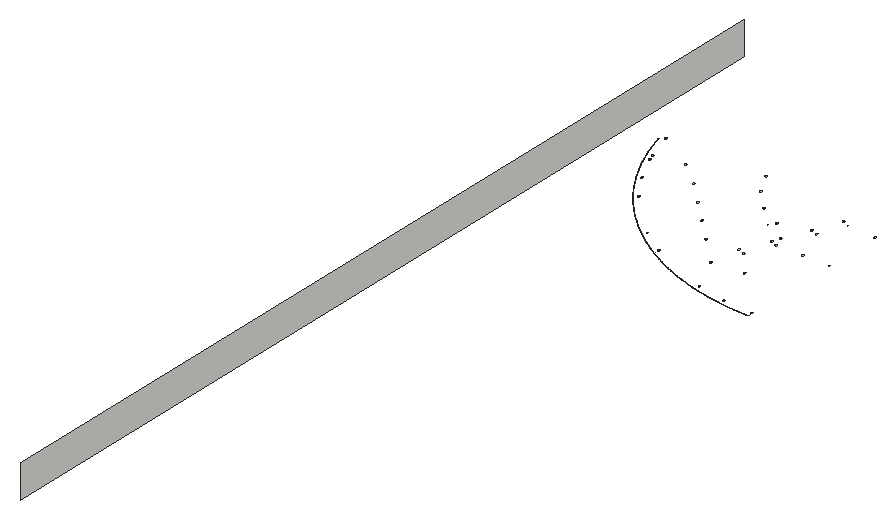
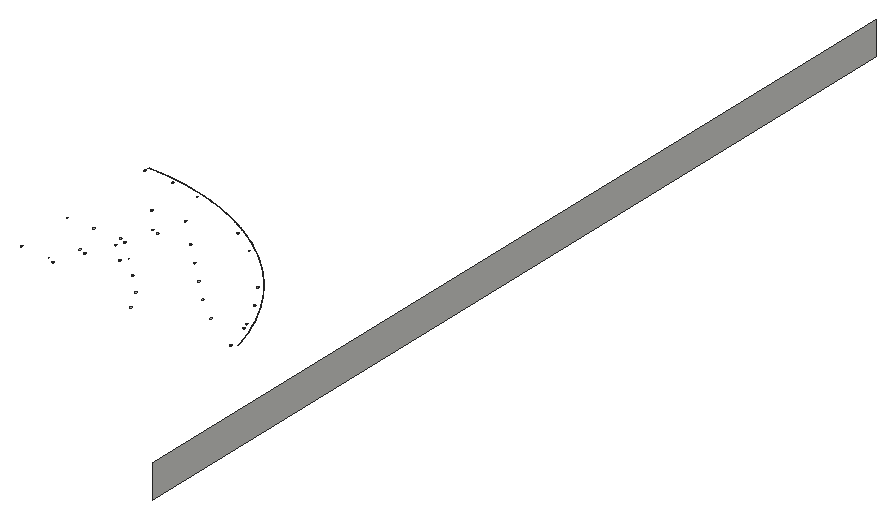
# SketchUp Ruby script. Lengths in inches.
U = 1.inch
M = Sketchup.active_model
def pt(a) = Geom::Point3d.new(a.map { |v| v * U })
def face(e, loops, mat)
  f = e.add_face(loops[0].map { |a| pt(a) })
  loops[1..].each { |l| e.add_face(l.map { |a| pt(a) }).erase! }
  f.material = f.back_material = mat if mat
  f
end
# faces: each face lists its corners as indices into pts; further lists are holes
def faces(e, pts, list, mat = nil) = list.each { |f| face(e, (f[0].is_a?(Array) ? f : [f]).map { |l| l.map { |i| pts[i] } }, mat) }
# xy, xz, yz: faces in a plane at the given z, y or x. An outline is a flat list of corners, or four numbers for a rectangle; further outlines are holes
def ring(l) = l.size == 4 ? [[l[0], l[1]], [l[2], l[1]], [l[2], l[3]], [l[0], l[3]]] : l.each_slice(2).to_a
def flat(e, list, mat, &to3) = list.each { |f| face(e, (f[0].is_a?(Array) ? f : [f]).map { |l| ring(l).map { |u, v| to3.(u, v) } }, mat) }
def xy(e, z, list, mat = nil) = flat(e, list, mat) { |x, y| [x, y, z] }
def xz(e, y, list, mat = nil) = flat(e, list, mat) { |x, z| [x, y, z] }
def yz(e, x, list, mat = nil) = flat(e, list, mat) { |y, z| [x, y, z] }
def lines(e, pts, list) = list.each { |a, b| e.add_line(pt(pts[a]), pt(pts[b])) }
# prism: a flat outline (further loops are holes) pulled along v
def prism(e, loops, v, mat = nil)
  f = face(e, loops, mat); d = Geom::Vector3d.new(v.map { |x| x * U })
  f.pushpull(f.normal.samedirection?(d) ? d.length : -d.length)
end
def box(e, o, s, mat = nil) = prism(e, [[o, [o[0] + s[0], o[1], o[2]], [o[0] + s[0], o[1] + s[1], o[2]], [o[0], o[1] + s[1], o[2]]]], [0, 0, s[2]], mat)
def at(x, y, z, deg = 0) = Geom::Transformation.translation(pt([x, y, z])) * Geom::Transformation.rotation(ORIGIN, Z_AXIS, deg.degrees)
def axes(o, x, y, z) = Geom::Transformation.new([*x, 0, *y, 0, *z, 0, *pt(o).to_a, 1])
def part(name) = M.definitions.add(name)
# library, detail: a bought-in or finely detailed component or shape, given as its bounding box
def library(name, o, s) = part(name).tap { |d| box(d.entities, o, s) }
def detail(e, o, s) = box(e.add_group.entities, o, s)
def put(e, d, t, mat = nil) = e.add_instance(d, t).tap { |i| i.material = mat if mat }
def group(e, t, mat = nil) = e.add_group.tap { |g| g.transformation = t; g.material = mat if mat }.entities
root = M.entities
M.materials.add("[Asphalt_Stamped_Brick]").color = [149, 133, 134]
M.materials.add("[Metal_Steel_Textured_White]").color = [191, 191, 191]
xy(root,3.625,[[146.528,137.349,146.523,137.35,146.518,137.352,146.514,137.355,146.511,137.359,146.509,137.364,146.508,137.369,146.509,137.374,146.511,137.379,146.514,137.383,146.518,137.387,146.523,137.389,146.533,137.389,146.538,137.387,146.542,137.383,146.545,137.379,146.547,137.374,146.548,137.369,146.547,137.364,146.545,137.359,146.542,137.355,146.538,137.352,146.533,137.35],[143.285,137.968,143.28,137.97,143.276,137.974,143.273,137.978,143.271,137.983,143.27,137.988,143.271,137.993,143.273,137.998,143.276,138.002,143.28,138.005,143.285,138.007,143.29,138.008,143.295,138.007,143.3,138.005,143.304,138.002,143.308,137.998,143.31,137.993,143.31,137.983,143.308,137.978,143.3,137.97,143.295,137.968],[136.475,140.789,136.47,140.791,136.466,140.794,136.463,140.799,136.461,140.803,136.46,140.809,136.461,140.814,136.463,140.819,136.466,140.823,136.47,140.826,136.475,140.828,136.486,140.828,136.49,140.826,136.495,140.823,136.498,140.819,136.5,140.814,136.5,140.803,136.498,140.799,136.495,140.794,136.49,140.791,136.486,140.789],[141.393,141.988,141.388,141.99,141.384,141.993,141.381,141.998,141.379,142.002,141.378,142.008,141.379,142.013,141.381,142.018,141.384,142.022,141.388,142.025,141.393,142.027,141.398,142.028,141.404,142.027,141.408,142.025,141.412,142.022,141.416,142.018,141.418,142.013,141.418,142.002,141.416,141.998,141.412,141.993,141.408,141.99,141.404,141.988],[144.852,142.332,144.847,142.333,144.842,142.335,144.838,142.338,144.834,142.342,144.832,142.347,144.832,142.357,144.834,142.362,144.838,142.366,144.842,142.369,144.847,142.371,144.852,142.372,144.857,142.371,144.862,142.369,144.866,142.366,144.869,142.362,144.871,142.357,144.872,142.352,144.871,142.347,144.869,142.342,144.866,142.338,144.862,142.335,144.857,142.333],
  [133.748,142.641,133.744,142.643,133.736,142.651,133.734,142.656,133.734,142.666,133.736,142.671,133.74,142.675,133.744,142.678,133.748,142.68,133.754,142.681,133.759,142.68,133.764,142.678,133.768,142.675,133.771,142.671,133.773,142.666,133.774,142.661,133.773,142.656,133.771,142.651,133.768,142.647,133.764,142.643,133.759,142.641],[129.101,147.293,129.096,147.294,129.091,147.296,129.087,147.299,129.084,147.303,129.082,147.308,129.081,147.313,129.082,147.318,129.084,147.323,129.087,147.327,129.091,147.33,129.096,147.332,129.101,147.333,129.106,147.332,129.111,147.33,129.115,147.327,129.118,147.323,129.12,147.318,129.121,147.313,129.12,147.308,129.118,147.303,129.115,147.299,129.111,147.296,129.106,147.294],[136.116,147.32,136.111,147.322,136.107,147.326,136.104,147.33,136.102,147.334,136.101,147.34,136.102,147.345,136.104,147.35,136.107,147.354,136.111,147.357,136.116,147.359,136.121,147.36,136.126,147.359,136.131,147.357,136.135,147.354,136.138,147.35,136.14,147.345,136.141,147.34,136.14,147.334,136.138,147.33,136.135,147.326,136.131,147.322,136.126,147.32],[143.146,148.293,143.141,148.294,143.136,148.296,143.132,148.299,143.129,148.303,143.127,148.308,143.126,148.313,143.127,148.318,143.129,148.323,143.132,148.327,143.136,148.33,143.141,148.332,143.146,148.333,143.151,148.332,143.156,148.33,143.16,148.327,143.163,148.323,143.165,148.318,143.166,148.313,143.165,148.308,143.163,148.303,143.16,148.299,143.156,148.296,143.151,148.294],[141.49,151.073,141.485,151.075,141.481,151.079,141.478,151.083,141.476,151.088,141.476,151.098,141.478,151.103,141.481,151.107,141.485,151.11,141.49,151.112,141.495,151.113,141.501,151.112,141.505,151.11,141.51,151.107,141.513,151.103,141.515,151.098,141.515,151.088,141.513,151.083,141.51,151.079,141.505,151.075,141.501,151.073],
  [144.679,151.995,144.674,151.996,144.669,151.998,144.665,152.001,144.662,152.005,144.66,152.01,144.659,152.015,144.66,152.02,144.662,152.025,144.665,152.029,144.669,152.033,144.674,152.035,144.685,152.035,144.689,152.033,144.694,152.029,144.697,152.025,144.699,152.02,144.699,152.01,144.697,152.005,144.694,152.001,144.689,151.998,144.685,151.996],[138.95,152.489,138.945,152.49,138.94,152.492,138.936,152.495,138.932,152.499,138.93,152.504,138.93,152.514,138.932,152.519,138.94,152.527,138.945,152.529,138.955,152.529,138.96,152.527,138.964,152.523,138.967,152.519,138.969,152.514,138.97,152.509,138.969,152.504,138.967,152.499,138.964,152.495,138.96,152.492,138.955,152.49],[125.749,152.958,125.744,152.96,125.74,152.963,125.736,152.968,125.734,152.972,125.734,152.983,125.736,152.988,125.74,152.992,125.744,152.995,125.749,152.997,125.754,152.998,125.759,152.997,125.764,152.995,125.768,152.992,125.771,152.988,125.773,152.983,125.774,152.978,125.773,152.972,125.771,152.968,125.768,152.963,125.764,152.96,125.759,152.958],[125.448,153.695,125.443,153.696,125.438,153.698,125.434,153.701,125.431,153.705,125.429,153.71,125.428,153.715,125.429,153.72,125.431,153.725,125.434,153.729,125.438,153.733,125.443,153.735,125.453,153.735,125.458,153.733,125.462,153.729,125.465,153.725,125.467,153.72,125.468,153.715,125.467,153.71,125.465,153.705,125.462,153.701,125.458,153.698,125.453,153.696],[145.882,154.899,145.877,154.9,145.872,154.902,145.868,154.905,145.865,154.909,145.863,154.914,145.862,154.919,145.863,154.924,145.865,154.929,145.868,154.933,145.872,154.936,145.877,154.938,145.882,154.939,145.887,154.938,145.892,154.936,145.896,154.933,145.9,154.929,145.902,154.924,145.902,154.914,145.9,154.909,145.896,154.905,145.892,154.902,145.887,154.9],
  [124.428,156.83,124.423,156.831,124.418,156.833,124.414,156.836,124.411,156.84,124.409,156.845,124.408,156.85,124.409,156.855,124.411,156.86,124.414,156.864,124.418,156.867,124.423,156.869,124.428,156.87,124.433,156.869,124.438,156.867,124.442,156.864,124.446,156.86,124.448,156.855,124.448,156.845,124.446,156.84,124.442,156.836,124.438,156.833,124.433,156.831]],"[Asphalt_Stamped_Brick]")
xy(root,3.625,[[149.818,137.073,149.795,137.076,149.773,137.085,149.755,137.099,149.741,137.118,149.732,137.139,149.729,137.162,149.732,137.185,149.741,137.207,149.755,137.225,149.773,137.239,149.795,137.248,149.818,137.251,149.818,137.25,149.795,137.247,149.774,137.238,149.756,137.224,149.742,137.206,149.733,137.185,149.73,137.162,149.733,137.139,149.742,137.118,149.756,137.1,149.774,137.086,149.795,137.077,149.818,137.074],[149.818,137.074,149.795,137.077,149.774,137.086,149.756,137.1,149.742,137.118,149.733,137.139,149.73,137.162,149.733,137.185,149.742,137.206,149.756,137.224,149.774,137.238,149.795,137.247,149.818,137.25,149.818,137.199,149.808,137.197,149.8,137.194,149.792,137.188,149.786,137.18,149.783,137.172,149.781,137.162,149.783,137.153,149.786,137.144,149.792,137.136,149.8,137.13,149.808,137.127,149.818,137.125],[149.818,137.125,149.808,137.127,149.8,137.13,149.792,137.136,149.786,137.144,149.783,137.153,149.781,137.162,149.783,137.172,149.786,137.18,149.792,137.188,149.8,137.194,149.808,137.197,149.818,137.199,149.818,137.182,149.813,137.181,149.808,137.179,149.804,137.176,149.801,137.172,149.799,137.167,149.798,137.162,149.799,137.157,149.801,137.152,149.804,137.148,149.808,137.145,149.813,137.143,149.818,137.142],[149.818,137.142,149.818,137.182,149.823,137.181,149.828,137.179,149.832,137.176,149.835,137.172,149.837,137.167,149.838,137.162,149.837,137.157,149.835,137.152,149.832,137.148,149.828,137.145,149.823,137.143],[[146.528,137.281,146.505,137.284,146.484,137.293,146.466,137.307,146.452,137.325,146.443,137.347,146.44,137.369,146.443,137.392,146.452,137.413,146.466,137.432,146.484,137.445,146.505,137.454,146.528,137.457,146.551,137.454,146.572,137.445,146.59,137.432,146.604,137.413,146.613,137.392,146.616,137.369,146.613,137.347,146.604,137.325,146.59,137.307,146.572,137.293,146.551,137.284],[146.528,137.333,146.538,137.334,146.546,137.338,146.554,137.343,146.56,137.351,146.563,137.36,146.565,137.369,146.563,137.379,146.56,137.388,146.554,137.395,146.546,137.401,146.538,137.405,146.528,137.406,146.519,137.405,146.51,137.401,146.502,137.395,146.496,137.388,146.493,137.379,146.491,137.369,146.493,137.36,146.496,137.351,146.502,137.343,146.51,137.338,146.519,137.334]],
  [[146.528,137.333,146.519,137.334,146.51,137.338,146.502,137.343,146.496,137.351,146.493,137.36,146.491,137.369,146.493,137.379,146.496,137.388,146.502,137.395,146.51,137.401,146.519,137.405,146.528,137.406,146.538,137.405,146.546,137.401,146.554,137.395,146.56,137.388,146.563,137.379,146.565,137.369,146.563,137.36,146.56,137.351,146.554,137.343,146.546,137.338,146.538,137.334],[146.528,137.349,146.533,137.35,146.538,137.352,146.542,137.355,146.545,137.359,146.547,137.364,146.548,137.369,146.547,137.374,146.545,137.379,146.542,137.383,146.538,137.387,146.533,137.389,146.523,137.389,146.518,137.387,146.514,137.383,146.511,137.379,146.509,137.374,146.508,137.369,146.509,137.364,146.511,137.359,146.514,137.355,146.518,137.352,146.523,137.35]],[[143.29,137.9,143.268,137.903,143.246,137.912,143.228,137.926,143.214,137.944,143.205,137.965,143.202,137.988,143.205,138.011,143.214,138.032,143.228,138.05,143.246,138.064,143.268,138.073,143.29,138.076,143.313,138.073,143.334,138.064,143.352,138.05,143.366,138.032,143.375,138.011,143.378,137.988,143.375,137.965,143.366,137.944,143.352,137.926,143.334,137.912,143.313,137.903],[143.29,137.951,143.3,137.952,143.309,137.956,143.316,137.962,143.322,137.969,143.326,137.978,143.327,137.988,143.326,137.997,143.322,138.006,143.316,138.014,143.309,138.019,143.3,138.023,143.29,138.024,143.281,138.023,143.272,138.019,143.264,138.014,143.259,138.006,143.255,137.997,143.254,137.988,143.255,137.978,143.259,137.969,143.264,137.962,143.272,137.956,143.281,137.952]],[[143.29,137.951,143.281,137.952,143.272,137.956,143.264,137.962,143.259,137.969,143.255,137.978,143.254,137.988,143.255,137.997,143.259,138.006,143.264,138.014,143.272,138.019,143.281,138.023,143.29,138.024,143.3,138.023,143.309,138.019,143.316,138.014,143.322,138.006,143.326,137.997,143.327,137.988,143.326,137.978,143.322,137.969,143.316,137.962,143.309,137.956,143.3,137.952],[143.285,137.968,143.295,137.968,143.3,137.97,143.308,137.978,143.31,137.983,143.31,137.993,143.308,137.998,143.304,138.002,143.3,138.005,143.295,138.007,143.29,138.008,143.285,138.007,143.28,138.005,143.276,138.002,143.273,137.998,143.271,137.993,143.27,137.988,143.271,137.983,143.273,137.978,143.276,137.974,143.28,137.97]],[[136.48,140.721,136.458,140.724,136.436,140.732,136.418,140.746,136.404,140.765,136.395,140.786,136.392,140.809,136.395,140.831,136.404,140.852,136.418,140.871,136.436,140.885,136.458,140.893,136.48,140.896,136.503,140.893,136.524,140.885,136.543,140.871,136.557,140.852,136.565,140.831,136.568,140.809,136.565,140.786,136.557,140.765,136.543,140.746,136.524,140.732,136.503,140.724],[136.48,140.772,136.49,140.773,136.499,140.777,136.506,140.783,136.512,140.79,136.516,140.799,136.517,140.809,136.516,140.818,136.512,140.827,136.506,140.834,136.499,140.84,136.49,140.844,136.48,140.845,136.471,140.844,136.462,140.84,136.455,140.834,136.449,140.827,136.445,140.818,136.444,140.809,136.445,140.799,136.449,140.79,136.455,140.783,136.462,140.777,136.471,140.773]],[[136.48,140.772,136.471,140.773,136.462,140.777,136.455,140.783,136.449,140.79,136.445,140.799,136.444,140.809,136.445,140.818,136.449,140.827,136.455,140.834,136.462,140.84,136.471,140.844,136.48,140.845,136.49,140.844,136.499,140.84,136.506,140.834,136.512,140.827,136.516,140.818,136.517,140.809,136.516,140.799,136.512,140.79,136.506,140.783,136.499,140.777,136.49,140.773],[136.475,140.789,136.486,140.789,136.49,140.791,136.495,140.794,136.498,140.799,136.5,140.803,136.5,140.814,136.498,140.819,136.495,140.823,136.49,140.826,136.486,140.828,136.475,140.828,136.47,140.826,136.466,140.823,136.463,140.819,136.461,140.814,136.46,140.809,136.461,140.803,136.463,140.799,136.466,140.794,136.47,140.791]],
  [[141.398,141.92,141.376,141.923,141.354,141.931,141.336,141.945,141.322,141.964,141.313,141.985,141.31,142.008,141.313,142.03,141.322,142.052,141.336,142.07,141.354,142.084,141.376,142.093,141.398,142.096,141.421,142.093,141.442,142.084,141.461,142.07,141.474,142.052,141.483,142.03,141.486,142.008,141.483,141.985,141.474,141.964,141.461,141.945,141.442,141.931,141.421,141.923],[141.398,141.971,141.408,141.972,141.417,141.976,141.424,141.982,141.43,141.989,141.434,141.998,141.435,142.008,141.434,142.017,141.43,142.026,141.424,142.033,141.417,142.039,141.408,142.043,141.398,142.044,141.389,142.043,141.38,142.039,141.372,142.033,141.367,142.026,141.363,142.017,141.362,142.008,141.363,141.998,141.367,141.989,141.372,141.982,141.38,141.976,141.389,141.972]],[[141.398,141.971,141.389,141.972,141.38,141.976,141.372,141.982,141.367,141.989,141.363,141.998,141.362,142.008,141.363,142.017,141.367,142.026,141.372,142.033,141.38,142.039,141.389,142.043,141.398,142.044,141.408,142.043,141.417,142.039,141.424,142.033,141.43,142.026,141.434,142.017,141.435,142.008,141.434,141.998,141.43,141.989,141.424,141.982,141.417,141.976,141.408,141.972],[141.393,141.988,141.404,141.988,141.408,141.99,141.412,141.993,141.416,141.998,141.418,142.002,141.418,142.013,141.416,142.018,141.412,142.022,141.408,142.025,141.404,142.027,141.398,142.028,141.393,142.027,141.388,142.025,141.384,142.022,141.381,142.018,141.379,142.013,141.378,142.008,141.379,142.002,141.381,141.998,141.384,141.993,141.388,141.99]],[[144.852,142.263,144.829,142.266,144.807,142.275,144.789,142.289,144.775,142.307,144.766,142.329,144.763,142.352,144.766,142.375,144.775,142.396,144.789,142.415,144.807,142.429,144.829,142.438,144.852,142.441,144.875,142.438,144.896,142.429,144.915,142.415,144.929,142.396,144.9375,142.375,144.941,142.352,144.9375,142.329,144.929,142.307,144.915,142.289,144.896,142.275,144.875,142.266],[144.852,142.264,144.874,142.267,144.896,142.276,144.914,142.29,144.928,142.308,144.937,142.329,144.94,142.352,144.937,142.375,144.928,142.396,144.914,142.414,144.896,142.428,144.874,142.437,144.852,142.44,144.829,142.437,144.808,142.428,144.79,142.414,144.776,142.396,144.767,142.375,144.764,142.352,144.767,142.329,144.776,142.308,144.79,142.29,144.808,142.276,144.829,142.267]],[[144.852,142.264,144.829,142.267,144.808,142.276,144.79,142.29,144.776,142.308,144.767,142.329,144.764,142.352,144.767,142.375,144.776,142.396,144.79,142.414,144.808,142.428,144.829,142.437,144.852,142.44,144.874,142.437,144.896,142.428,144.914,142.414,144.928,142.396,144.937,142.375,144.94,142.352,144.937,142.329,144.928,142.308,144.914,142.29,144.896,142.276,144.874,142.267],[144.852,142.315,144.861,142.317,144.87,142.32,144.878,142.326,144.883,142.334,144.887,142.342,144.888,142.352,144.887,142.361,144.883,142.37,144.878,142.378,144.87,142.384,144.861,142.387,144.852,142.389,144.842,142.387,144.833,142.384,144.826,142.378,144.82,142.37,144.816,142.361,144.815,142.352,144.816,142.342,144.82,142.334,144.826,142.326,144.833,142.32,144.842,142.317]],[[144.852,142.315,144.842,142.317,144.833,142.32,144.826,142.326,144.82,142.334,144.816,142.342,144.815,142.352,144.816,142.361,144.82,142.37,144.826,142.378,144.833,142.384,144.842,142.387,144.852,142.389,144.861,142.387,144.87,142.384,144.878,142.378,144.883,142.37,144.887,142.361,144.888,142.352,144.887,142.342,144.883,142.334,144.878,142.326,144.87,142.32,144.861,142.317],[144.852,142.332,144.857,142.333,144.862,142.335,144.866,142.338,144.869,142.342,144.871,142.347,144.872,142.352,144.871,142.357,144.869,142.362,144.866,142.366,144.862,142.369,144.857,142.371,144.852,142.372,144.847,142.371,144.842,142.369,144.838,142.366,144.834,142.362,144.832,142.357,144.832,142.347,144.834,142.342,144.838,142.338,144.842,142.335,144.847,142.333]],
  [[133.754,142.624,133.744,142.625,133.735,142.629,133.728,142.635,133.722,142.642,133.718,142.651,133.717,142.661,133.718,142.67,133.722,142.679,133.728,142.687,133.735,142.692,133.744,142.696,133.754,142.697,133.763,142.696,133.772,142.692,133.78,142.687,133.785,142.679,133.789,142.67,133.79,142.661,133.789,142.651,133.785,142.642,133.78,142.635,133.772,142.629,133.763,142.625],[133.748,142.641,133.759,142.641,133.764,142.643,133.768,142.647,133.771,142.651,133.773,142.656,133.774,142.661,133.773,142.666,133.771,142.671,133.768,142.675,133.764,142.678,133.759,142.68,133.754,142.681,133.748,142.68,133.744,142.678,133.74,142.675,133.736,142.671,133.734,142.666,133.734,142.656,133.736,142.651,133.744,142.643]],[[138.462,144.911,138.439,144.914,138.418,144.922,138.4,144.936,138.386,144.955,138.377,144.976,138.374,144.999,138.377,145.021,138.386,145.043,138.4,145.061,138.418,145.075,138.439,145.083,138.462,145.086,138.485,145.083,138.506,145.075,138.524,145.061,138.538,145.043,138.547,145.021,138.55,144.999,138.547,144.976,138.538,144.955,138.524,144.936,138.506,144.922,138.485,144.914],[138.462,144.962,138.472,144.963,138.481,144.967,138.488,144.973,138.494,144.98,138.498,144.989,138.499,144.999,138.498,145.008,138.494,145.017,138.488,145.024,138.481,145.03,138.472,145.034,138.462,145.035,138.453,145.034,138.444,145.03,138.436,145.024,138.431,145.017,138.427,145.008,138.426,144.999,138.427,144.989,138.431,144.98,138.436,144.973,138.444,144.967,138.453,144.963]],[[142.641,144.919,142.618,144.922,142.597,144.931,142.578,144.945,142.564,144.963,142.555,144.985,142.552,145.008,142.555,145.031,142.564,145.052,142.578,145.07,142.597,145.085,142.618,145.093,142.641,145.096,142.664,145.093,142.685,145.085,142.704,145.07,142.718,145.052,142.727,145.031,142.73,145.008,142.727,144.985,142.718,144.963,142.704,144.945,142.685,144.931,142.664,144.922],[142.641,144.92,142.664,144.923,142.685,144.931,142.703,144.945,142.717,144.964,142.726,144.985,142.729,145.008,142.726,145.03,142.717,145.052,142.703,145.07,142.685,145.084,142.664,145.092,142.641,145.095,142.618,145.092,142.597,145.084,142.579,145.07,142.565,145.052,142.556,145.03,142.553,145.008,142.556,144.985,142.565,144.964,142.579,144.945,142.597,144.931,142.618,144.923]],[[138.462,144.962,138.453,144.963,138.444,144.967,138.436,144.973,138.431,144.98,138.427,144.989,138.426,144.999,138.427,145.008,138.431,145.017,138.436,145.024,138.444,145.03,138.453,145.034,138.462,145.035,138.472,145.034,138.481,145.03,138.488,145.024,138.494,145.017,138.498,145.008,138.499,144.999,138.498,144.989,138.494,144.98,138.488,144.973,138.481,144.967,138.472,144.963],[138.457,144.979,138.467,144.979,138.472,144.981,138.476,144.984,138.48,144.989,138.482,144.993,138.482,145.004,138.48,145.009,138.476,145.013,138.472,145.016,138.467,145.018,138.462,145.019,138.457,145.018,138.452,145.016,138.448,145.013,138.445,145.009,138.443,145.004,138.442,144.999,138.443,144.993,138.445,144.989,138.448,144.984,138.452,144.981]],[[141.903,145.224,141.88,145.227,141.859,145.236,141.84,145.25,141.826,145.269,141.817,145.29,141.814,145.313,141.817,145.336,141.826,145.358,141.84,145.376,141.859,145.39,141.88,145.399,141.903,145.402,141.926,145.399,141.948,145.39,141.966,145.376,141.98,145.358,141.989,145.336,141.992,145.313,141.989,145.29,141.98,145.269,141.966,145.25,141.948,145.236,141.926,145.227],[141.903,145.225,141.926,145.228,141.947,145.237,141.965,145.251,141.979,145.269,141.988,145.29,141.991,145.313,141.988,145.336,141.979,145.357,141.965,145.375,141.947,145.389,141.926,145.398,141.903,145.401,141.881,145.398,141.859,145.389,141.841,145.375,141.827,145.357,141.818,145.336,141.815,145.313,141.818,145.29,141.827,145.269,141.841,145.251,141.859,145.237,141.881,145.228]],
  [[129.101,147.224,129.078,147.227,129.057,147.236,129.038,147.25,129.024,147.269,129.015,147.29,129.012,147.313,129.015,147.336,129.024,147.358,129.038,147.376,129.057,147.39,129.078,147.399,129.101,147.402,129.124,147.399,129.146,147.39,129.164,147.376,129.178,147.358,129.187,147.336,129.19,147.313,129.187,147.29,129.178,147.269,129.164,147.25,129.146,147.236,129.124,147.227],[129.101,147.225,129.124,147.228,129.145,147.237,129.163,147.251,129.177,147.269,129.186,147.29,129.189,147.313,129.186,147.336,129.177,147.357,129.163,147.375,129.145,147.389,129.124,147.398,129.101,147.401,129.078,147.398,129.057,147.389,129.039,147.375,129.025,147.357,129.016,147.336,129.013,147.313,129.016,147.29,129.025,147.269,129.039,147.251,129.057,147.237,129.078,147.228]],[[136.121,147.252,136.098,147.255,136.077,147.263,136.059,147.277,136.045,147.296,136.036,147.317,136.033,147.34,136.036,147.362,136.045,147.384,136.059,147.402,136.077,147.416,136.098,147.425,136.121,147.428,136.144,147.425,136.165,147.416,136.183,147.402,136.197,147.384,136.206,147.362,136.209,147.34,136.206,147.317,136.197,147.296,136.183,147.277,136.165,147.263,136.144,147.255],[136.121,147.303,136.131,147.304,136.139,147.308,136.147,147.314,136.153,147.321,136.157,147.33,136.158,147.34,136.157,147.349,136.153,147.358,136.147,147.365,136.139,147.371,136.131,147.375,136.121,147.376,136.112,147.375,136.103,147.371,136.095,147.365,136.089,147.358,136.086,147.349,136.085,147.34,136.086,147.33,136.089,147.321,136.095,147.314,136.103,147.308,136.112,147.304]],[[129.101,147.277,129.092,147.278,129.083,147.281,129.075,147.287,129.069,147.295,129.066,147.304,129.065,147.313,129.066,147.323,129.069,147.331,129.075,147.339,129.083,147.345,129.092,147.349,129.101,147.35,129.111,147.349,129.119,147.345,129.127,147.339,129.133,147.331,129.137,147.323,129.138,147.313,129.137,147.304,129.133,147.295,129.127,147.287,129.119,147.281,129.111,147.278],[129.101,147.293,129.106,147.294,129.111,147.296,129.115,147.299,129.118,147.303,129.12,147.308,129.121,147.313,129.12,147.318,129.118,147.323,129.115,147.327,129.111,147.33,129.106,147.332,129.101,147.333,129.096,147.332,129.091,147.33,129.087,147.327,129.084,147.323,129.082,147.318,129.081,147.313,129.082,147.308,129.084,147.303,129.087,147.299,129.091,147.296,129.096,147.294]],[[136.121,147.303,136.112,147.304,136.103,147.308,136.095,147.314,136.089,147.321,136.086,147.33,136.085,147.34,136.086,147.349,136.089,147.358,136.095,147.365,136.103,147.371,136.112,147.375,136.121,147.376,136.131,147.375,136.139,147.371,136.147,147.365,136.153,147.358,136.157,147.349,136.158,147.34,136.157,147.33,136.153,147.321,136.147,147.314,136.139,147.308,136.131,147.304],[136.116,147.32,136.126,147.32,136.131,147.322,136.135,147.326,136.138,147.33,136.14,147.334,136.141,147.34,136.14,147.345,136.138,147.35,136.135,147.354,136.131,147.357,136.126,147.359,136.121,147.36,136.116,147.359,136.111,147.357,136.107,147.354,136.104,147.35,136.102,147.345,136.101,147.34,136.102,147.334,136.104,147.33,136.107,147.326,136.111,147.322]],[[143.884,147.919,143.861,147.922,143.839,147.931,143.821,147.945,143.807,147.963,143.798,147.985,143.795,148.008,143.798,148.031,143.807,148.052,143.821,148.07,143.839,148.085,143.861,148.093,143.884,148.096,143.907,148.093,143.928,148.085,143.946,148.07,143.961,148.052,143.969,148.031,143.972,148.008,143.969,147.985,143.961,147.963,143.946,147.945,143.928,147.931,143.907,147.922],[143.884,147.92,143.906,147.923,143.928,147.931,143.946,147.945,143.96,147.964,143.969,147.985,143.972,148.008,143.969,148.03,143.96,148.051,143.946,148.07,143.928,148.084,143.906,148.092,143.884,148.095,143.861,148.092,143.84,148.084,143.821,148.07,143.807,148.051,143.799,148.03,143.796,148.008,143.799,147.985,143.807,147.964,143.821,147.945,143.84,147.931,143.861,147.923]],
  [[146.851,147.919,146.828,147.922,146.806,147.931,146.788,147.945,146.774,147.963,146.765,147.985,146.762,148.008,146.765,148.031,146.774,148.052,146.788,148.07,146.806,148.085,146.828,148.093,146.851,148.096,146.874,148.093,146.895,148.085,146.914,148.07,146.928,148.052,146.937,148.031,146.94,148.008,146.937,147.985,146.928,147.963,146.914,147.945,146.895,147.931,146.874,147.922],[146.851,147.92,146.873,147.923,146.895,147.931,146.913,147.945,146.927,147.964,146.936,147.985,146.939,148.008,146.936,148.03,146.927,148.051,146.913,148.07,146.895,148.084,146.873,148.092,146.851,148.095,146.828,148.092,146.807,148.084,146.789,148.07,146.775,148.051,146.766,148.03,146.763,148.008,146.766,147.985,146.775,147.964,146.789,147.945,146.807,147.931,146.828,147.923]],[149.818,147.971,149.808,147.972,149.8,147.976,149.792,147.982,149.786,147.989,149.783,147.998,149.781,148.008,149.783,148.017,149.786,148.026,149.792,148.033,149.8,148.039,149.808,148.043,149.818,148.044,149.818,148.027,149.813,148.027,149.808,148.025,149.804,148.022,149.801,148.018,149.799,148.013,149.798,148.008,149.799,148.002,149.801,147.998,149.804,147.993,149.808,147.99,149.813,147.988,149.818,147.988],[[143.146,148.224,143.123,148.227,143.101,148.236,143.083,148.25,143.069,148.269,143.06,148.29,143.057,148.313,143.06,148.336,143.069,148.358,143.083,148.376,143.101,148.39,143.123,148.399,143.146,148.402,143.169,148.399,143.19,148.39,143.209,148.376,143.223,148.358,143.232,148.336,143.235,148.313,143.232,148.29,143.223,148.269,143.209,148.25,143.19,148.236,143.169,148.227],[143.146,148.225,143.169,148.228,143.19,148.237,143.208,148.251,143.222,148.269,143.231,148.29,143.234,148.313,143.231,148.336,143.222,148.357,143.208,148.375,143.19,148.389,143.169,148.398,143.146,148.401,143.123,148.398,143.102,148.389,143.084,148.375,143.07,148.357,143.061,148.336,143.058,148.313,143.061,148.29,143.07,148.269,143.084,148.251,143.102,148.237,143.123,148.228]],[[143.146,148.276,143.136,148.278,143.128,148.281,143.12,148.287,143.114,148.295,143.111,148.304,143.109,148.313,143.111,148.323,143.114,148.331,143.12,148.339,143.128,148.345,143.136,148.348,143.146,148.35,143.155,148.348,143.164,148.345,143.172,148.339,143.178,148.331,143.181,148.323,143.183,148.313,143.181,148.304,143.178,148.295,143.172,148.287,143.164,148.281,143.155,148.278],[143.146,148.293,143.151,148.294,143.156,148.296,143.16,148.299,143.163,148.303,143.165,148.308,143.166,148.313,143.165,148.318,143.163,148.323,143.16,148.327,143.156,148.33,143.151,148.332,143.146,148.333,143.141,148.332,143.136,148.33,143.132,148.327,143.129,148.323,143.127,148.318,143.126,148.313,143.127,148.308,143.129,148.303,143.132,148.299,143.136,148.296,143.141,148.294]],[[143.477,149.024,143.454,149.027,143.433,149.035,143.414,149.049,143.401,149.068,143.392,149.089,143.389,149.112,143.392,149.134,143.401,149.155,143.414,149.174,143.433,149.1875,143.454,149.196,143.477,149.199,143.499,149.196,143.521,149.1875,143.539,149.174,143.553,149.155,143.562,149.134,143.565,149.112,143.562,149.089,143.553,149.068,143.539,149.049,143.521,149.035,143.499,149.027],[143.477,149.075,143.486,149.076,143.495,149.08,143.503,149.086,143.508,149.093,143.512,149.102,143.513,149.112,143.512,149.121,143.508,149.13,143.503,149.137,143.495,149.143,143.486,149.147,143.477,149.148,143.467,149.147,143.458,149.143,143.451,149.137,143.445,149.13,143.441,149.121,143.44,149.112,143.441,149.102,143.445,149.093,143.451,149.086,143.458,149.08,143.467,149.076]],
  [[143.477,149.075,143.467,149.076,143.458,149.08,143.451,149.086,143.445,149.093,143.441,149.102,143.44,149.112,143.441,149.121,143.445,149.13,143.451,149.137,143.458,149.143,143.467,149.147,143.477,149.148,143.486,149.147,143.495,149.143,143.503,149.137,143.508,149.13,143.512,149.121,143.513,149.112,143.512,149.102,143.508,149.093,143.503,149.086,143.495,149.08,143.486,149.076],[143.471,149.092,143.482,149.092,143.487,149.094,143.491,149.097,143.494,149.102,143.496,149.106,143.497,149.112,143.496,149.117,143.494,149.121,143.491,149.126,143.487,149.129,143.482,149.131,143.471,149.131,143.467,149.129,143.463,149.126,143.459,149.121,143.457,149.117,143.457,149.106,143.459,149.102,143.463,149.097,143.467,149.094]],[143.471,149.092,143.467,149.094,143.463,149.097,143.459,149.102,143.457,149.106,143.457,149.117,143.459,149.121,143.463,149.126,143.467,149.129,143.471,149.131,143.482,149.131,143.487,149.129,143.491,149.126,143.494,149.121,143.496,149.117,143.497,149.112,143.496,149.106,143.494,149.102,143.491,149.097,143.487,149.094,143.482,149.092],[[133.78,149.592,133.757,149.595,133.736,149.604,133.717,149.618,133.703,149.636,133.694,149.658,133.691,149.681,133.694,149.704,133.703,149.725,133.717,149.744,133.736,149.758,133.757,149.767,133.78,149.77,133.803,149.767,133.825,149.758,133.843,149.744,133.857,149.725,133.866,149.704,133.869,149.681,133.866,149.658,133.857,149.636,133.843,149.618,133.825,149.604,133.803,149.595],[133.78,149.593,133.803,149.596,133.824,149.605,133.842,149.619,133.856,149.637,133.865,149.658,133.868,149.681,133.865,149.703,133.856,149.725,133.842,149.743,133.824,149.757,133.803,149.766,133.78,149.769,133.757,149.766,133.736,149.757,133.718,149.743,133.704,149.725,133.695,149.703,133.692,149.681,133.695,149.658,133.704,149.637,133.718,149.619,133.736,149.605,133.757,149.596]],[[127.249,149.952,127.226,149.955,127.205,149.964,127.187,149.978,127.173,149.996,127.164,150.017,127.161,150.04,127.164,150.0625,127.173,150.084,127.187,150.102,127.205,150.116,127.226,150.125,127.249,150.128,127.272,150.125,127.293,150.116,127.311,150.102,127.325,150.084,127.334,150.0625,127.337,150.04,127.334,150.017,127.325,149.996,127.311,149.978,127.293,149.964,127.272,149.955],[127.249,150.003,127.258,150.005,127.267,150.008,127.275,150.014,127.281,150.022,127.284,150.03,127.286,150.04,127.284,150.049,127.281,150.058,127.275,150.066,127.267,150.072,127.258,150.075,127.249,150.077,127.24,150.075,127.231,150.072,127.223,150.066,127.217,150.058,127.214,150.049,127.212,150.04,127.214,150.03,127.217,150.022,127.223,150.014,127.231,150.008,127.24,150.005]],[[127.249,150.003,127.24,150.005,127.231,150.008,127.223,150.014,127.217,150.022,127.214,150.03,127.212,150.04,127.214,150.049,127.217,150.058,127.223,150.066,127.231,150.072,127.24,150.075,127.249,150.077,127.258,150.075,127.267,150.072,127.275,150.066,127.281,150.058,127.284,150.049,127.286,150.04,127.284,150.03,127.281,150.022,127.275,150.014,127.267,150.008,127.258,150.005],[127.249,150.02,127.254,150.021,127.259,150.023,127.263,150.026,127.266,150.03,127.268,150.035,127.269,150.04,127.268,150.045,127.266,150.05,127.263,150.054,127.259,150.057,127.254,150.059,127.249,150.06,127.244,150.059,127.239,150.057,127.235,150.054,127.232,150.05,127.23,150.045,127.229,150.04,127.23,150.035,127.232,150.03,127.235,150.026,127.239,150.023,127.244,150.021]],
  [141.048,150.391,141.043,150.392,141.038,150.394,141.034,150.397,141.031,150.401,141.029,150.406,141.028,150.411,141.029,150.416,141.031,150.421,141.034,150.425,141.038,150.428,141.043,150.43,141.048,150.431,141.053,150.43,141.058,150.428,141.062,150.425,141.065,150.421,141.067,150.416,141.068,150.411,141.067,150.406,141.065,150.401,141.062,150.397,141.058,150.394,141.053,150.392],[[141.495,151.004,141.472,151.007,141.451,151.016,141.433,151.03,141.418,151.048,141.41,151.07,141.407,151.093,141.41,151.116,141.418,151.137,141.433,151.156,141.451,151.17,141.472,151.179,141.495,151.182,141.518,151.179,141.54,151.17,141.558,151.156,141.572,151.137,141.581,151.116,141.584,151.093,141.581,151.07,141.572,151.048,141.558,151.03,141.54,151.016,141.518,151.007],[141.495,151.005,141.518,151.008,141.539,151.017,141.558,151.03,141.572,151.049,141.58,151.07,141.583,151.093,141.58,151.115,141.572,151.137,141.558,151.155,141.539,151.169,141.518,151.178,141.495,151.181,141.473,151.178,141.452,151.169,141.433,151.155,141.419,151.137,141.411,151.115,141.408,151.093,141.411,151.07,141.419,151.049,141.433,151.03,141.452,151.017,141.473,151.008]],[[141.495,151.005,141.473,151.008,141.452,151.017,141.433,151.03,141.419,151.049,141.411,151.07,141.408,151.093,141.411,151.115,141.419,151.137,141.433,151.155,141.452,151.169,141.473,151.178,141.495,151.181,141.518,151.178,141.539,151.169,141.558,151.155,141.572,151.137,141.58,151.115,141.583,151.093,141.58,151.07,141.572,151.049,141.558,151.03,141.539,151.017,141.518,151.008],[141.495,151.056,141.505,151.057,141.514,151.061,141.521,151.067,141.527,151.074,141.531,151.083,141.532,151.093,141.531,151.102,141.527,151.111,141.521,151.119,141.514,151.124,141.505,151.128,141.495,151.129,141.486,151.128,141.477,151.124,141.47,151.119,141.464,151.111,141.46,151.102,141.459,151.093,141.46,151.083,141.464,151.074,141.47,151.067,141.477,151.061,141.486,151.057]],[[141.495,151.056,141.486,151.057,141.477,151.061,141.47,151.067,141.464,151.074,141.46,151.083,141.459,151.093,141.46,151.102,141.464,151.111,141.47,151.119,141.477,151.124,141.486,151.128,141.495,151.129,141.505,151.128,141.514,151.124,141.521,151.119,141.527,151.111,141.531,151.102,141.532,151.093,141.531,151.083,141.527,151.074,141.521,151.067,141.514,151.061,141.505,151.057],[141.49,151.073,141.501,151.073,141.505,151.075,141.51,151.079,141.513,151.083,141.515,151.088,141.515,151.098,141.513,151.103,141.51,151.107,141.505,151.11,141.501,151.112,141.495,151.113,141.49,151.112,141.485,151.11,141.481,151.107,141.478,151.103,141.476,151.098,141.476,151.088,141.478,151.083,141.481,151.079,141.485,151.075]],[[145.417,151.622,145.394,151.625,145.373,151.634,145.355,151.648,145.341,151.666,145.332,151.687,145.329,151.71,145.332,151.733,145.341,151.754,145.355,151.772,145.373,151.786,145.394,151.795,145.417,151.798,145.44,151.795,145.461,151.786,145.479,151.772,145.493,151.754,145.502,151.733,145.505,151.71,145.502,151.687,145.493,151.666,145.479,151.648,145.461,151.634,145.44,151.625],[145.417,151.673,145.427,151.674,145.435,151.678,145.443,151.684,145.449,151.691,145.452,151.7,145.454,151.71,145.452,151.719,145.449,151.728,145.443,151.736,145.435,151.741,145.427,151.745,145.417,151.746,145.408,151.745,145.399,151.741,145.391,151.736,145.385,151.728,145.382,151.719,145.38,151.71,145.382,151.7,145.385,151.691,145.391,151.684,145.399,151.678,145.408,151.674]],
  [[144.679,151.927,144.657,151.93,144.635,151.939,144.617,151.953,144.603,151.971,144.595,151.993,144.592,152.015,144.595,152.038,144.603,152.059,144.617,152.077,144.635,152.091,144.657,152.1,144.679,152.103,144.702,152.1,144.723,152.091,144.742,152.077,144.756,152.059,144.764,152.038,144.767,152.015,144.764,151.993,144.756,151.971,144.742,151.953,144.723,151.939,144.702,151.93],[144.679,151.979,144.689,151.98,144.698,151.984,144.705,151.989,144.711,151.997,144.715,152.006,144.716,152.015,144.715,152.025,144.711,152.034,144.705,152.041,144.698,152.047,144.689,152.051,144.679,152.052,144.67,152.051,144.661,152.047,144.654,152.041,144.648,152.034,144.644,152.025,144.643,152.015,144.644,152.006,144.648,151.997,144.654,151.989,144.661,151.984,144.67,151.98]],[[131.439,151.933,131.416,151.936,131.395,151.945,131.376,151.959,131.362,151.977,131.353,151.999,131.35,152.022,131.353,152.045,131.362,152.066,131.376,152.085,131.395,152.099,131.416,152.108,131.439,152.111,131.462,152.108,131.483,152.099,131.502,152.085,131.516,152.066,131.525,152.045,131.528,152.022,131.525,151.999,131.516,151.977,131.502,151.959,131.483,151.945,131.462,151.936],[131.439,151.934,131.462,151.937,131.483,151.946,131.501,151.96,131.515,151.978,131.524,151.999,131.527,152.022,131.524,152.045,131.515,152.066,131.501,152.084,131.483,152.098,131.462,152.107,131.439,152.11,131.416,152.107,131.395,152.098,131.377,152.084,131.363,152.066,131.354,152.045,131.351,152.022,131.354,151.999,131.363,151.978,131.377,151.96,131.395,151.946,131.416,151.937]],[[144.679,151.979,144.67,151.98,144.661,151.984,144.654,151.989,144.648,151.997,144.644,152.006,144.643,152.015,144.644,152.025,144.648,152.034,144.654,152.041,144.661,152.047,144.67,152.051,144.679,152.052,144.689,152.051,144.698,152.047,144.705,152.041,144.711,152.034,144.715,152.025,144.716,152.015,144.715,152.006,144.711,151.997,144.705,151.989,144.698,151.984,144.689,151.98],[144.679,151.995,144.685,151.996,144.689,151.998,144.694,152.001,144.697,152.005,144.699,152.01,144.699,152.02,144.697,152.025,144.694,152.029,144.689,152.033,144.685,152.035,144.674,152.035,144.669,152.033,144.665,152.029,144.662,152.025,144.66,152.02,144.659,152.015,144.66,152.01,144.662,152.005,144.665,152.001,144.669,151.998,144.674,151.996]],[[138.95,152.421,138.927,152.424,138.906,152.433,138.888,152.447,138.874,152.465,138.865,152.487,138.862,152.509,138.865,152.532,138.874,152.553,138.888,152.571,138.906,152.585,138.927,152.594,138.95,152.597,138.972,152.594,138.994,152.585,139.012,152.571,139.026,152.553,139.035,152.532,139.038,152.509,139.035,152.487,139.026,152.465,139.012,152.447,138.994,152.433,138.972,152.424],[138.95,152.473,138.959,152.474,138.968,152.478,138.976,152.483,138.981,152.491,138.985,152.5,138.986,152.509,138.985,152.519,138.981,152.528,138.976,152.535,138.968,152.541,138.959,152.545,138.95,152.546,138.94,152.545,138.931,152.541,138.924,152.535,138.918,152.528,138.914,152.519,138.913,152.509,138.914,152.5,138.918,152.491,138.924,152.483,138.931,152.478,138.94,152.474]],[[138.95,152.473,138.94,152.474,138.931,152.478,138.924,152.483,138.918,152.491,138.914,152.5,138.913,152.509,138.914,152.519,138.918,152.528,138.924,152.535,138.931,152.541,138.94,152.545,138.95,152.546,138.959,152.545,138.968,152.541,138.976,152.535,138.981,152.528,138.985,152.519,138.986,152.509,138.985,152.5,138.981,152.491,138.976,152.483,138.968,152.478,138.959,152.474],[138.95,152.489,138.955,152.49,138.96,152.492,138.964,152.495,138.967,152.499,138.969,152.504,138.97,152.509,138.969,152.514,138.967,152.519,138.964,152.523,138.96,152.527,138.955,152.529,138.945,152.529,138.94,152.527,138.932,152.519,138.93,152.514,138.93,152.504,138.932,152.499,138.936,152.495,138.94,152.492,138.945,152.49]],
  [[125.754,152.889,125.731,152.892,125.709,152.901,125.691,152.915,125.677,152.933,125.668,152.955,125.665,152.978,125.668,153.001,125.677,153.022,125.691,153.04,125.709,153.055,125.731,153.063,125.754,153.066,125.777,153.063,125.798,153.055,125.817,153.04,125.831,153.022,125.84,153.001,125.843,152.978,125.84,152.955,125.831,152.933,125.817,152.915,125.798,152.901,125.777,152.892],[125.754,152.89,125.776,152.893,125.798,152.901,125.816,152.915,125.83,152.934,125.839,152.955,125.842,152.978,125.839,153,125.83,153.022,125.816,153.04,125.798,153.054,125.776,153.0625,125.754,153.066,125.731,153.0625,125.71,153.054,125.691,153.04,125.678,153.022,125.669,153,125.666,152.978,125.669,152.955,125.678,152.934,125.691,152.915,125.71,152.901,125.731,152.893]],[[125.754,152.89,125.731,152.893,125.71,152.901,125.691,152.915,125.678,152.934,125.669,152.955,125.666,152.978,125.669,153,125.678,153.022,125.691,153.04,125.71,153.054,125.731,153.0625,125.754,153.066,125.776,153.0625,125.798,153.054,125.816,153.04,125.83,153.022,125.839,153,125.842,152.978,125.839,152.955,125.83,152.934,125.816,152.915,125.798,152.901,125.776,152.893],[125.754,152.941,125.763,152.942,125.772,152.946,125.78,152.952,125.785,152.959,125.789,152.968,125.79,152.978,125.789,152.987,125.785,152.996,125.78,153.003,125.772,153.009,125.763,153.013,125.754,153.014,125.744,153.013,125.735,153.009,125.728,153.003,125.722,152.996,125.718,152.987,125.717,152.978,125.718,152.968,125.722,152.959,125.728,152.952,125.735,152.946,125.744,152.942]],[[125.754,152.941,125.744,152.942,125.735,152.946,125.728,152.952,125.722,152.959,125.718,152.968,125.717,152.978,125.718,152.987,125.722,152.996,125.728,153.003,125.735,153.009,125.744,153.013,125.754,153.014,125.763,153.013,125.772,153.009,125.78,153.003,125.785,152.996,125.789,152.987,125.79,152.978,125.789,152.968,125.785,152.959,125.78,152.952,125.772,152.946,125.763,152.942],[125.749,152.958,125.759,152.958,125.764,152.96,125.768,152.963,125.771,152.968,125.773,152.972,125.774,152.978,125.773,152.983,125.771,152.988,125.768,152.992,125.764,152.995,125.759,152.997,125.754,152.998,125.749,152.997,125.744,152.995,125.74,152.992,125.736,152.988,125.734,152.983,125.734,152.972,125.736,152.968,125.74,152.963,125.744,152.96]],[[125.448,153.627,125.425,153.63,125.404,153.639,125.386,153.653,125.372,153.671,125.363,153.692,125.36,153.715,125.363,153.738,125.372,153.759,125.386,153.777,125.404,153.791,125.425,153.8,125.448,153.803,125.471,153.8,125.492,153.791,125.51,153.777,125.524,153.759,125.533,153.738,125.536,153.715,125.533,153.692,125.524,153.671,125.51,153.653,125.492,153.639,125.471,153.63],[125.448,153.679,125.458,153.68,125.466,153.684,125.474,153.689,125.48,153.697,125.483,153.706,125.485,153.715,125.483,153.725,125.48,153.734,125.474,153.741,125.466,153.747,125.458,153.751,125.448,153.752,125.439,153.751,125.43,153.747,125.422,153.741,125.416,153.734,125.413,153.725,125.412,153.715,125.413,153.706,125.416,153.697,125.422,153.689,125.43,153.684,125.439,153.68]],[[125.448,153.679,125.439,153.68,125.43,153.684,125.422,153.689,125.416,153.697,125.413,153.706,125.412,153.715,125.413,153.725,125.416,153.734,125.422,153.741,125.43,153.747,125.439,153.751,125.448,153.752,125.458,153.751,125.466,153.747,125.474,153.741,125.48,153.734,125.483,153.725,125.485,153.715,125.483,153.706,125.48,153.697,125.474,153.689,125.466,153.684,125.458,153.68],[125.448,153.695,125.453,153.696,125.458,153.698,125.462,153.701,125.465,153.705,125.467,153.71,125.468,153.715,125.467,153.72,125.465,153.725,125.462,153.729,125.458,153.733,125.453,153.735,125.443,153.735,125.438,153.733,125.434,153.729,125.431,153.725,125.429,153.72,125.428,153.715,125.429,153.71,125.431,153.705,125.434,153.701,125.438,153.698,125.443,153.696]],
  [[128.754,154.131,128.731,154.134,128.709,154.143,128.691,154.157,128.677,154.176,128.668,154.197,128.665,154.22,128.668,154.243,128.677,154.265,128.691,154.283,128.709,154.297,128.731,154.306,128.754,154.309,128.777,154.306,128.798,154.297,128.816,154.283,128.831,154.265,128.839,154.243,128.843,154.22,128.839,154.197,128.831,154.176,128.816,154.157,128.798,154.143,128.777,154.134],[128.754,154.132,128.776,154.135,128.798,154.144,128.816,154.158,128.83,154.176,128.839,154.197,128.842,154.22,128.839,154.243,128.83,154.264,128.816,154.282,128.798,154.296,128.776,154.305,128.754,154.308,128.731,154.305,128.71,154.296,128.691,154.282,128.677,154.264,128.669,154.243,128.666,154.22,128.669,154.197,128.677,154.176,128.691,154.158,128.71,154.144,128.731,154.135]],[[149.818,154.373,149.818,154.374,149.795,154.377,149.774,154.385,149.756,154.399,149.742,154.418,149.733,154.439,149.73,154.462,149.733,154.484,149.742,154.506,149.756,154.524,149.774,154.538,149.795,154.546,149.818,154.549,149.818,154.55,149.841,154.547,149.862,154.539,149.881,154.524,149.895,154.506,149.904,154.485,149.907,154.462,149.904,154.439,149.895,154.417,149.881,154.399,149.862,154.385,149.841,154.376],[149.818,154.425,149.818,154.442,149.813,154.442,149.808,154.444,149.804,154.447,149.801,154.452,149.799,154.456,149.798,154.462,149.799,154.467,149.801,154.472,149.804,154.476,149.808,154.479,149.813,154.481,149.818,154.482,149.818,154.498,149.808,154.497,149.8,154.493,149.792,154.487,149.786,154.48,149.783,154.471,149.781,154.462,149.783,154.452,149.786,154.443,149.792,154.436,149.8,154.43,149.808,154.426],[149.818,154.442,149.823,154.442,149.828,154.444,149.832,154.447,149.835,154.452,149.837,154.456,149.838,154.462,149.837,154.467,149.835,154.472,149.832,154.476,149.828,154.479,149.823,154.481,149.818,154.482]],[149.818,154.425,149.808,154.426,149.8,154.43,149.792,154.436,149.786,154.443,149.783,154.452,149.781,154.462,149.783,154.471,149.786,154.48,149.792,154.487,149.8,154.493,149.808,154.497,149.818,154.498,149.818,154.482,149.813,154.481,149.808,154.479,149.804,154.476,149.801,154.472,149.799,154.467,149.798,154.462,149.799,154.456,149.801,154.452,149.804,154.447,149.808,154.444,149.813,154.442,149.818,154.442],[[136.852,154.518,136.829,154.521,136.807,154.53,136.789,154.545,136.775,154.563,136.766,154.584,136.763,154.607,136.766,154.63,136.775,154.652,136.789,154.67,136.807,154.684,136.829,154.693,136.852,154.696,136.875,154.693,136.896,154.684,136.914,154.67,136.929,154.652,136.9375,154.63,136.941,154.607,136.9375,154.584,136.929,154.563,136.914,154.545,136.896,154.53,136.875,154.521],[136.852,154.519,136.874,154.522,136.896,154.531,136.914,154.545,136.928,154.563,136.937,154.585,136.94,154.607,136.937,154.63,136.928,154.651,136.914,154.67,136.896,154.684,136.874,154.692,136.852,154.695,136.829,154.692,136.808,154.684,136.789,154.67,136.775,154.651,136.767,154.63,136.764,154.607,136.767,154.585,136.775,154.563,136.789,154.545,136.808,154.531,136.829,154.522]],[[146.62,154.577,146.61,154.578,146.602,154.582,146.594,154.588,146.588,154.595,146.585,154.604,146.583,154.614,146.585,154.623,146.588,154.632,146.594,154.639,146.602,154.645,146.61,154.649,146.62,154.65,146.629,154.649,146.638,154.645,146.646,154.639,146.652,154.632,146.655,154.623,146.656,154.614,146.655,154.604,146.652,154.595,146.646,154.588,146.638,154.582,146.629,154.578],[146.615,154.594,146.625,154.594,146.63,154.596,146.634,154.599,146.637,154.604,146.639,154.608,146.64,154.614,146.639,154.619,146.637,154.624,146.634,154.628,146.63,154.631,146.625,154.633,146.615,154.633,146.61,154.631,146.606,154.628,146.603,154.624,146.601,154.619,146.6,154.614,146.601,154.608,146.603,154.604,146.606,154.599,146.61,154.596]],
  [146.615,154.594,146.61,154.596,146.606,154.599,146.603,154.604,146.601,154.608,146.6,154.614,146.601,154.619,146.603,154.624,146.606,154.628,146.61,154.631,146.615,154.633,146.625,154.633,146.63,154.631,146.634,154.628,146.637,154.624,146.639,154.619,146.64,154.614,146.639,154.608,146.637,154.604,146.634,154.599,146.63,154.596,146.625,154.594],[[145.882,154.831,145.859,154.834,145.838,154.843,145.82,154.857,145.806,154.875,145.797,154.896,145.794,154.919,145.797,154.942,145.806,154.963,145.82,154.981,145.838,154.995,145.859,155.004,145.882,155.007,145.905,155.004,145.926,154.995,145.944,154.981,145.958,154.963,145.967,154.942,145.97,154.919,145.967,154.896,145.958,154.875,145.944,154.857,145.926,154.843,145.905,154.834],[145.882,154.882,145.892,154.884,145.901,154.887,145.908,154.893,145.914,154.901,145.918,154.91,145.919,154.919,145.918,154.929,145.914,154.9375,145.908,154.945,145.901,154.951,145.892,154.954,145.882,154.956,145.873,154.954,145.864,154.951,145.856,154.945,145.851,154.9375,145.847,154.929,145.846,154.919,145.847,154.91,145.851,154.901,145.856,154.893,145.864,154.887,145.873,154.884]],[[145.882,154.882,145.873,154.884,145.864,154.887,145.856,154.893,145.851,154.901,145.847,154.91,145.846,154.919,145.847,154.929,145.851,154.9375,145.856,154.945,145.864,154.951,145.873,154.954,145.882,154.956,145.892,154.954,145.901,154.951,145.908,154.945,145.914,154.9375,145.918,154.929,145.919,154.919,145.918,154.91,145.914,154.901,145.908,154.893,145.901,154.887,145.892,154.884],[145.882,154.899,145.887,154.9,145.892,154.902,145.896,154.905,145.9,154.909,145.902,154.914,145.902,154.924,145.9,154.929,145.896,154.933,145.892,154.936,145.887,154.938,145.882,154.939,145.877,154.938,145.872,154.936,145.868,154.933,145.865,154.929,145.863,154.924,145.862,154.919,145.863,154.914,145.865,154.909,145.868,154.905,145.872,154.902,145.877,154.9]],[[124.428,156.761,124.405,156.764,124.384,156.773,124.365,156.787,124.351,156.805,124.342,156.827,124.339,156.85,124.342,156.873,124.351,156.894,124.365,156.913,124.384,156.927,124.405,156.936,124.428,156.939,124.451,156.936,124.473,156.927,124.491,156.913,124.505,156.894,124.514,156.873,124.517,156.85,124.514,156.827,124.505,156.805,124.491,156.787,124.473,156.773,124.451,156.764],[124.428,156.762,124.451,156.765,124.472,156.774,124.49,156.788,124.504,156.806,124.513,156.827,124.516,156.85,124.513,156.873,124.504,156.894,124.49,156.912,124.472,156.926,124.451,156.935,124.428,156.938,124.405,156.935,124.384,156.926,124.366,156.912,124.352,156.894,124.343,156.873,124.34,156.85,124.343,156.827,124.352,156.806,124.366,156.788,124.384,156.774,124.405,156.765]],[[124.428,156.762,124.405,156.765,124.384,156.774,124.366,156.788,124.352,156.806,124.343,156.827,124.34,156.85,124.343,156.873,124.352,156.894,124.366,156.912,124.384,156.926,124.405,156.935,124.428,156.938,124.451,156.935,124.472,156.926,124.49,156.912,124.504,156.894,124.513,156.873,124.516,156.85,124.513,156.827,124.504,156.806,124.49,156.788,124.472,156.774,124.451,156.765],[124.428,156.813,124.438,156.814,124.447,156.818,124.454,156.824,124.46,156.832,124.464,156.84,124.465,156.85,124.464,156.859,124.46,156.868,124.454,156.876,124.447,156.882,124.438,156.885,124.428,156.886,124.419,156.885,124.41,156.882,124.402,156.876,124.397,156.868,124.393,156.859,124.392,156.85,124.393,156.84,124.397,156.832,124.402,156.824,124.41,156.818,124.419,156.814]],
  [[124.428,156.813,124.419,156.814,124.41,156.818,124.402,156.824,124.397,156.832,124.393,156.84,124.392,156.85,124.393,156.859,124.397,156.868,124.402,156.876,124.41,156.882,124.419,156.885,124.428,156.886,124.438,156.885,124.447,156.882,124.454,156.876,124.46,156.868,124.464,156.859,124.465,156.85,124.464,156.84,124.46,156.832,124.454,156.824,124.447,156.818,124.438,156.814],[124.428,156.83,124.433,156.831,124.438,156.833,124.442,156.836,124.446,156.84,124.448,156.845,124.448,156.855,124.446,156.86,124.442,156.864,124.438,156.867,124.433,156.869,124.428,156.87,124.423,156.869,124.418,156.867,124.414,156.864,124.411,156.86,124.409,156.855,124.408,156.85,124.409,156.845,124.411,156.84,124.414,156.836,124.418,156.833,124.423,156.831]],[[135.552,156.948,135.529,156.951,135.508,156.96,135.49,156.974,135.476,156.992,135.467,157.013,135.464,157.036,135.467,157.059,135.476,157.08,135.49,157.098,135.508,157.112,135.529,157.121,135.552,157.124,135.575,157.121,135.596,157.112,135.614,157.098,135.628,157.08,135.637,157.059,135.64,157.036,135.637,157.013,135.628,156.992,135.614,156.974,135.596,156.96,135.575,156.951],[135.552,157,135.561,157.001,135.57,157.004,135.578,157.01,135.584,157.018,135.587,157.027,135.589,157.036,135.587,157.046,135.584,157.054,135.578,157.062,135.57,157.068,135.561,157.072,135.552,157.073,135.543,157.072,135.534,157.068,135.526,157.062,135.52,157.054,135.517,157.046,135.515,157.036,135.517,157.027,135.52,157.018,135.526,157.01,135.534,157.004,135.543,157.001]]],"[Metal_Steel_Textured_White]")
yz(root,116.615,[[76.29,0,177.536,3.625]])
p = [[149.818,136.63,3.625],[149.818,136.563,3.625],[127.908,148.036,3.625],[129.328,146.184,3.625],[130.904,144.464,3.625],[132.625,142.888,3.625],
  [134.476,141.467,3.625],[136.444,140.213,3.625],[136.411,140.156,3.625],[138.486,139.076,3.625],[140.647,138.18,3.625],[142.878,137.477,3.625],
  [145.162,136.971,3.625],[147.481,136.665,3.625],[126.654,150.004,3.625],[136.511,140.329,3.625],[140.67,138.243,3.625],[142.895,137.541,3.625],
  [145.173,137.036,3.625],[147.487,136.732,3.625],[123.917,156.4375,3.625],[124.621,154.206,3.625],[125.516,152.045,3.625],[126.596,149.97,3.625],
  [127.853,147.997,3.625],[129.277,146.142,3.625],[130.857,144.417,3.625],[123.982,156.455,3.625],[124.683,154.229,3.625],[125.576,152.073,3.625],
  [132.582,142.837,3.625],[134.438,141.413,3.625],[138.514,139.136,3.625],[149.818,136.763,3.625]]
lines(root,p,[[0,1],[2,3],[3,4],[4,5],[5,6],[6,7],[8,7],[8,9],[9,10],[10,11],[11,12],[12,13],
  [13,1],[14,2],[7,15],[16,17],[17,18],[18,19],[19,0],[20,21],[21,22],[22,23],[23,24],[24,25],
  [25,26],[27,28],[28,29],[29,14],[26,30],[30,31],[31,8],[7,32],[32,16],[33,0]])
